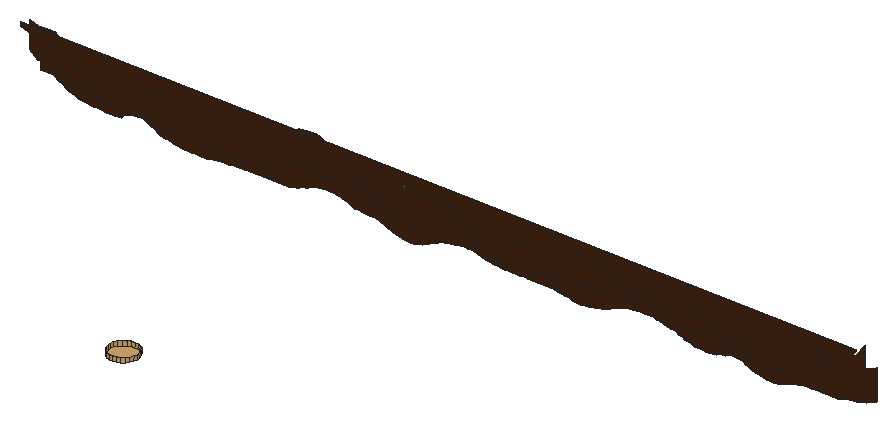
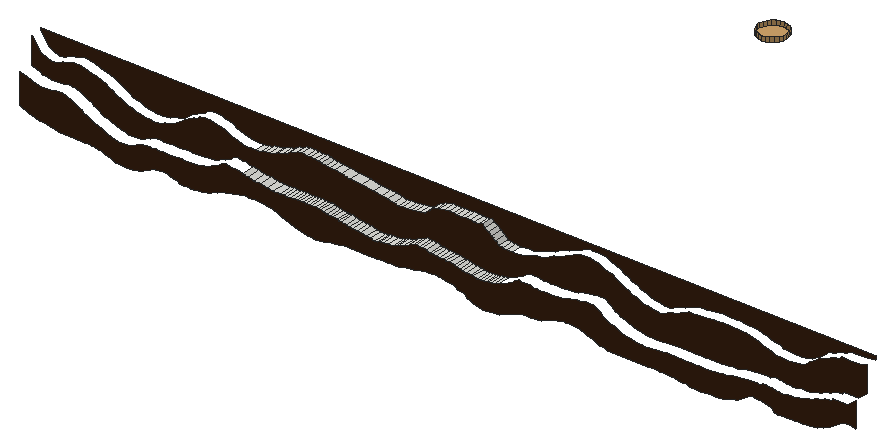
# SketchUp Ruby script. Lengths in inches.
U = 1.inch
M = Sketchup.active_model
def pt(a) = Geom::Point3d.new(a.map { |v| v * U })
def face(e, loops, mat)
  f = e.add_face(loops[0].map { |a| pt(a) })
  loops[1..].each { |l| e.add_face(l.map { |a| pt(a) }).erase! }
  f.material = f.back_material = mat if mat
  f
end
# faces: each face lists its corners as indices into pts; further lists are holes
def faces(e, pts, list, mat = nil) = list.each { |f| face(e, (f[0].is_a?(Array) ? f : [f]).map { |l| l.map { |i| pts[i] } }, mat) }
# xy, xz, yz: faces in a plane at the given z, y or x. An outline is a flat list of corners, or four numbers for a rectangle; further outlines are holes
def ring(l) = l.size == 4 ? [[l[0], l[1]], [l[2], l[1]], [l[2], l[3]], [l[0], l[3]]] : l.each_slice(2).to_a
def flat(e, list, mat, &to3) = list.each { |f| face(e, (f[0].is_a?(Array) ? f : [f]).map { |l| ring(l).map { |u, v| to3.(u, v) } }, mat) }
def xy(e, z, list, mat = nil) = flat(e, list, mat) { |x, y| [x, y, z] }
def xz(e, y, list, mat = nil) = flat(e, list, mat) { |x, z| [x, y, z] }
def yz(e, x, list, mat = nil) = flat(e, list, mat) { |y, z| [x, y, z] }
def lines(e, pts, list) = list.each { |a, b| e.add_line(pt(pts[a]), pt(pts[b])) }
# prism: a flat outline (further loops are holes) pulled along v
def prism(e, loops, v, mat = nil)
  f = face(e, loops, mat); d = Geom::Vector3d.new(v.map { |x| x * U })
  f.pushpull(f.normal.samedirection?(d) ? d.length : -d.length)
end
def box(e, o, s, mat = nil) = prism(e, [[o, [o[0] + s[0], o[1], o[2]], [o[0] + s[0], o[1] + s[1], o[2]], [o[0], o[1] + s[1], o[2]]]], [0, 0, s[2]], mat)
def at(x, y, z, deg = 0) = Geom::Transformation.translation(pt([x, y, z])) * Geom::Transformation.rotation(ORIGIN, Z_AXIS, deg.degrees)
def axes(o, x, y, z) = Geom::Transformation.new([*x, 0, *y, 0, *z, 0, *pt(o).to_a, 1])
def part(name) = M.definitions.add(name)
# library, detail: a bought-in or finely detailed component or shape, given as its bounding box
def library(name, o, s) = part(name).tap { |d| box(d.entities, o, s) }
def detail(e, o, s) = box(e.add_group.entities, o, s)
def put(e, d, t, mat = nil) = e.add_instance(d, t).tap { |i| i.material = mat if mat }
def group(e, t, mat = nil) = e.add_group.tap { |g| g.transformation = t; g.material = mat if mat }.entities
root = M.entities
M.materials.add("[Field Square Tile]").color = [211, 167, 108]
M.materials.add("[Wood Veneer 01]").color = [66, 38, 20]
xy(root,243.05,[[2115.79,2398.8,2116.47,2401.37]])
xy(root,243.07,[[2113.9375,2398.8,2114.52,2401.37]])
xy(root,243.09,[[2110.625,2398.8,2111.15,2401.37],[2111.15,2398.8,2111.67,2401.37],[2111.67,2398.8,2112.33,2401.37],[2112.33,2398.8,2112.78,2401.37]])
xy(root,249.21,[[2083.42,2396.68,2084.31,2398.8]])
xy(root,249.22,[[2085.03,2396.68,2085.9375,2398.8]])
xy(root,249.23,[[2086.58,2396.68,2087.48,2398.8]])
xy(root,250.6875,[[2081.97,2328.39,2081.31,2328.48,2080.69,2328.74,2080.16,2329.14,2079.75,2329.68,2079.5,2330.29,2079.41,2330.96,2079.5,2331.62,2079.75,2332.24,2080.16,2332.77,2080.69,2333.18,2081.31,2333.43,2081.97,2333.52,2082.63,2333.43,2083.25,2333.18,2083.78,2332.77,2084.19,2332.24,2084.45,2331.62,2084.53,2330.96,2084.45,2330.29,2084.19,2329.68,2083.78,2329.14,2083.25,2328.74,2082.63,2328.48]],"[Field Square Tile]")
xz(root,2396.68,[[2141.84,244.87,2142.75,245.01,2143.6875,245.12,2144.45,245.25,2145.21,245.41,2145.84,245.78,2146.64,245.88,2147.35,246.16,2147.95,246.57,2148.74,246.9,2149.34,247.35,2150.01,247.62,2150.6,248.06,2151.36,248.32,2152.47,248.66,2153.25,248.79,2154.11,249.19,2154.78,249.32,2155.71,249.41,2156.56,249.48,2157.31,249.21,2157.95,248.96,2158.65,248.9,2159.45,248.42,2160.16,248.3,2160.87,248.22,2161.6875,248.56,2162.62,249.02,2164.35,251.16,2164.35,251.5,2010.34,251.5,2010.34,250.88,2011.93,250.53,2013.55,250.54,2015.01,250.55,2015.54,250.15,2016.15,249.97,2016.95,249.8,2017.62,249.41,2018.29,249.2,2019.06,249.01,2019.55,248.51,2020.18,248.07,2020.83,247.72,2021.47,247.25,2022.02,246.88,2022.74,246.73,2023.4,246.62,2024.14,246.54,2024.92,246.51,2025.7,246.58,2026.5,246.59,2027.3,246.69,2028.01,247.03,2028.7,247.2,2029.67,247.39,2030.3,247.78,2031.08,247.89,2032.08,248.18,2032.72,248.29,2033.61,248.35,2034.34,248.4,2035.33,248.4375,2035.99,248.46,2036.88,248.47,2037.62,248.48,2038.51,248.49,2039.24,248.39,2040.64,248.28,2041.67,248.15,2042.49,248.11,2043.29,248.08,2044.13,247.66,2044.76,247.46,2045.44,247.08,2046.125,246.94,2046.98,246.66,2047.59,246.35,2048.36,246.05,2049.26,246.13,2049.97,246.29,2050.77,246.41,2051.68,246.55,2052.41,246.92,2053.02,247.12,2053.7,247.31,2054.27,247.71,2055.2,248.03,2055.91,248.46,2056.69,248.82,2057.41,249.37,2058.2,249.5625,2059.1,249.9,2060.02,250.35,2060.68,250.49,2061.49,250.6,2062.51,250.58,2063.15,250.61,2063.77,250.32,2064.46,250.0625,2065.12,249.68,2065.88,249.46,2066.77,248.95,2067.99,248.69,2068.9,248.26,2069.5,247.9,2070.63,247.66,2071.21,247.53,2071.89,247.25,2072.7,246.95,2073.39,246.75,2074.18,246.66,2074.89,246.59,2075.78,246.55,2076.71,246.63,2077.45,246.74,2078.18,246.87,2078.79,247.42,2079.46,247.96,2080.03,248.44,2080.77,248.85,2081.24,249.34,2081.97,249.125,2082.74,249.17,2083.42,249.21,2084.31,249.21,2085.03,249.22,2085.9375,249.22,2086.58,249.23,2087.48,249.23,2088.22,249.24,2089.02,249.14,2089.65,248.82,2090.44,248.54,2091.14,248.04,2091.83,247.48,2092.72,247.29,2093.54,247.15,2094.27,247.05,2094.99,247,2095.9,246.96,2096.625,246.94,2097.54,247.04,2098.6,247.36,2099.78,247.43,2101.43,247.6,2103.41,247.98,2105.61,248.1875,2107.22,248.49,2108.47,248.62,2109.41,248.69,2110.09,248.75,2110.75,249.09,2111.45,249.18,2112.23,249.13,2112.93,249.17,2113.63,249.18,2114.53,249.29,2115.26,249.21,2115.87,248.8,2116.5625,248.73,2117.34,248.26,2118.04,248.02,2118.84,247.8125,2119.55,247.4,2120.46,247.27,2121.2,247.18,2122.125,246.91,2122.99,246.84,2123.94,246.79,2124.72,246.75,2125.47,246.83,2126.51,247.25,2127.38,247.55,2128.05,247.66,2128.68,248.16,2129.47,248.41,2130.17,248.52,2130.87,248.72,2131.57,248.8,2132.46,248.85,2133.29,248.6875,2133.83,248.26,2134.52,248.06,2135.41,247.55,2136.12,247.19,2136.93,246.63,2137.5625,246.13,2138.15,245.83,2138.83,245.67,2139.7,245.46,2140.41,245.0625,2141.125,244.95]],"[Wood Veneer 01]")
xz(root,2398.8,[[2145.84,241.09,2146.41,241.14,2147.05,241.35,2147.64,241.46,2148.58,241.85,2149.58,242.23,2150.14,242.42,2150.86,242.61,2151.375,242.91,2151.75,243.14,2152.29,243.52,2152.77,243.71,2153.1,244.02,2153.54,244.21,2154.13,244.57,2154.6,244.76,2155.22,245.125,2155.72,245.32,2156.2,245.41,2156.75,245.48,2157.24,245.59,2157.77,245.55,2158.38,245.35,2158.87,245.31,2159.42,245.27,2159.98,245.24,2160.54,245.22,2161.1,245.34,2161.73,245.42,2162.3125,245.52,2162.69,245.76,2163.16,245.9,2164.35,246.43,2164.35,251.16,2162.62,249.02,2161.6875,248.56,2160.87,248.22,2160.16,248.3,2159.45,248.42,2158.65,248.9,2157.95,248.96,2157.31,249.21,2156.56,249.48,2155.71,249.41,2154.78,249.32,2154.11,249.19,2153.25,248.79,2152.47,248.66,2151.36,248.32,2150.6,248.06,2150.01,247.62,2149.34,247.35,2148.74,246.9,2147.95,246.57,2147.35,246.16,2146.64,245.88,2145.84,245.78,2145.21,245.41,2144.45,245.25,2143.6875,245.12,2142.75,245.01,2141.84,244.87,2141.125,244.95,2140.41,245.0625,2139.7,245.46,2138.83,245.67,2138.15,245.83,2137.5625,246.13,2136.93,246.63,2136.12,247.19,2135.41,247.55,2134.52,248.06,2133.83,248.26,2133.29,248.6875,2132.46,248.85,2131.57,248.8,2130.87,248.72,2130.17,248.52,2129.47,248.41,2128.68,248.16,2128.05,247.66,2127.38,247.55,2126.51,247.25,2125.47,246.83,2124.72,246.75,2123.94,246.79,2122.99,246.84,2122.125,246.91,2121.2,247.18,2120.46,247.27,2119.55,247.4,2118.84,247.8125,2118.04,248.02,2117.34,248.26,2116.5625,248.73,2115.87,248.8,2115.26,249.21,2114.53,249.29,2113.63,249.18,2112.93,249.17,2112.23,249.13,2111.45,249.18,2110.75,249.09,2110.09,248.75,2109.41,248.69,2108.47,248.62,2107.22,248.49,2105.61,248.1875,2103.41,247.98,2101.43,247.6,2099.78,247.43,2098.6,247.36,2097.54,247.04,2096.625,246.94,2095.9,246.96,2094.99,247,2094.27,247.05,2093.54,247.15,2092.72,247.29,2091.83,247.48,2091.14,248.04,2090.44,248.54,2089.65,248.82,2089.02,249.14,2088.22,249.24,2087.48,249.23,2086.58,249.23,2085.9375,249.22,2085.03,249.22,2084.31,249.21,2083.42,249.21,2082.74,249.17,2081.97,249.125,2081.24,249.34,2080.77,248.85,2080.03,248.44,2079.46,247.96,2078.79,247.42,2078.18,246.87,2077.45,246.74,2076.71,246.63,2075.78,246.55,2074.89,246.59,2074.18,246.66,2073.39,246.75,2072.7,246.95,2071.89,247.25,2071.21,247.53,2070.63,247.66,2069.5,247.9,2068.9,248.26,2067.99,248.69,2066.77,248.95,2065.88,249.46,2065.12,249.68,2064.46,250.0625,2063.77,250.32,2063.15,250.61,2062.51,250.58,2061.49,250.6,2060.68,250.49,2060.02,250.35,2059.1,249.9,2058.2,249.5625,2057.41,249.37,2056.69,248.82,2055.91,248.46,2055.2,248.03,2054.27,247.71,2053.7,247.31,2053.02,247.12,2052.41,246.92,2051.68,246.55,2050.77,246.41,2049.97,246.29,2049.26,246.13,2048.36,246.05,2047.59,246.35,2046.98,246.66,2046.125,246.94,2045.44,247.08,2044.76,247.46,2044.13,247.66,2043.29,248.08,2042.49,248.11,2041.67,248.15,2040.64,248.28,2039.24,248.39,2038.51,248.49,2037.62,248.48,2036.88,248.47,2035.99,248.46,2035.33,248.4375,2034.34,248.4,2033.61,248.35,2032.72,248.29,2032.08,248.18,2031.08,247.89,2030.3,247.78,2029.67,247.39,2028.7,247.2,2028.01,247.03,2027.3,246.69,2026.5,246.59,2025.7,246.58,2024.92,246.51,2024.14,246.54,2023.4,246.62,2022.74,246.73,2022.02,246.88,2021.47,247.25,2020.83,247.72,2020.18,248.07,2019.55,248.51,2019.06,249.01,2018.29,249.2,2017.62,249.41,2016.95,249.8,2016.15,249.97,2015.54,250.15,2015.01,250.55,2013.55,250.54,2011.93,250.53,2010.34,250.88,2010.34,246.2,2011.91,244.96,2013.3,244.9375,2014.55,244.92,2014.77,244.61,2015.33,244.54,2016.09,244.41,2016.76,244.11,2017.28,243.95,2017.94,243.79,2018.46,243.48,2019.1,243.3,2019.6875,243.14,2020.17,243.06,2020.89,242.85,2021.47,242.78,2022.28,242.73,2022.82,242.68,2023.49,242.51,2024.01,242.46,2024.55,242.58,2025.18,242.57,2025.81,242.81,2026.38,242.86,2026.94,242.89,2027.58,242.92,2028.01,242.625,2028.62,242.65,2029.17,242.62,2029.8,242.58,2030.36,242.57,2031,242.48,2031.66,242.38,2032.32,242.34,2032.99,242.24,2034.16,241.96,2034.93,241.89,2035.75,241.83,2036.35,241.78,2037.12,241.75,2037.57,241.74,2038.12,241.72,2039.38,241.7,2040.11,241.69,2040.78,241.68,2041.37,241.68,2041.86,241.67,2042.5625,241.74,2043.13,241.75,2045.13,241.75,2045.62,241.67,2046.15,241.66,2046.76,241.57,2047.3,241.53,2047.92,241.51,2048.47,241.49,2049.17,241.48,2049.83,241.47,2050.4,241.46,2051.11,241.6,2051.84,241.85,2052.51,241.91,2053.41,242.1,2054.18,242.46,2054.88,242.78,2055.65,242.97,2056.18,243.23,2056.58,243.48,2057.1,243.72,2057.4375,244.12,2057.91,244.39,2058.39,244.73,2058.875,244.87,2059.46,244.95,2060.14,245.01,2060.79,244.81,2061.36,244.7,2061.84,244.67,2062.45,244.55,2062.99,244.51,2063.45,244.25,2064.2,244.11,2064.76,244.04,2065.38,243.99,2066.1,243.95,2066.6,243.93,2067.29,243.91,2067.86,243.89,2068.56,243.88,2069.21,243.94,2069.85,243.95,2070.41,244.1,2071.04,244.13,2071.52,244.15,2072.04,244.17,2072.56,244.18,2073.16,243.8,2073.7,243.43,2074.31,243.09,2074.7,242.875,2075.2,242.68,2075.79,242.51,2076.3,242.21,2076.9,242.11,2077.58,241.96,2078.14,241.89,2078.6,241.85,2079.12,241.8125,2079.63,241.79,2080.21,241.78,2080.88,241.91,2081.35,241.93,2082.02,242.09,2082.79,242.2,2083.29,242.24,2083.9,242.42,2084.45,242.47,2085.2,242.71,2085.84,242.78,2086.32,242.82,2087.01,242.85,2087.71,242.87,2088.26,243.02,2088.88,243.05,2089.43,243.29,2090.11,243.35,2090.66,243.39,2091.26,243.42,2092.03,243.14,2092.6,242.9375,2093.15,242.65,2093.77,242.39,2094.53,242.14,2095.17,241.89,2095.66,241.78,2096.71,241.63,2097.48,241.56,2098.08,241.51,2098.53,241.48,2099.05,241.46,2099.92,241.51,2100.64,241.59,2101.58,241.82,2102.36,241.87,2103.125,241.98,2103.74,242.02,2104.39,242.19,2105.09,242.38,2105.58,242.4375,2106.1,242.48,2106.76,242.58,2107.29,242.61,2107.875,242.77,2108.33,242.95,2108.89,243.01,2109.4,243.05,2109.97,243.08,2110.625,243.09,2112.78,243.09,2113.35,243.08,2113.9375,243.07,2114.52,243.07,2115.18,243.0625,2115.79,243.05,2116.47,243.05,2117.74,243.1,2118.91,243.17,2120.05,243.4,2121.3125,243.52,2122.44,243.71,2123.34,243.99,2124.04,244.08,2124.74,244.21,2125.32,244.27,2125.86,244.3,2126.53,244.39,2127.125,244.19,2127.5,243.88,2127.98,243.59,2128.53,243.33,2129.08,243.22,2129.57,242.92,2130.05,242.75,2130.61,242.6,2131.17,242.52,2131.73,242.47,2132.3125,242.43,2132.89,242.4,2133.47,242.39,2134.05,242.37,2134.63,242.36,2135.22,242.35,2136.38,242.33,2136.96,242.33,2137.68,242.32,2138.15,242.3125,2138.79,242.3,2139.46,242.3,2139.91,242.29,2140.55,242.28,2141.0625,242.28,2141.69,242.2,2142.27,241.97,2142.84,241.84,2143.35,241.57,2143.77,241.33,2144.24,241.24,2144.77,241.17,2145.24,241.12]],"[Wood Veneer 01]")
xz(root,2401.37,[[2079.2,236.98,2079.88,237.22,2080.73,237.43,2081.35,237.74,2082.05,238.02,2082.49,238.375,2083.05,238.51,2083.6875,238.76,2084.33,239.12,2084.91,239.22,2085.91,239.31,2086.72,239.54,2087.21,239.6,2087.83,239.65,2088.42,239.69,2088.98,239.7,2089.71,239.72,2090.32,239.56,2090.99,239.44,2091.84,239.16,2092.39,239.07,2093.16,238.93,2094.04,238.78,2094.52,238.73,2095.19,238.6875,2095.88,238.66,2096.55,238.65,2097.33,238.64,2097.95,238.63,2098.64,238.625,2099.5,238.625,2100.06,238.62,2104.95,238.62,2105.64,238.45,2106.4,238.25,2107.02,238.19,2107.79,238.15,2108.42,237.86,2109.19,237.79,2109.9,237.74,2110.77,237.87,2111.42,237.88,2112.54,238.14,2113.76,238.46,2114.51,238.72,2115.39,239.08,2116.18,239.375,2116.92,239.75,2117.57,239.97,2118.19,240.17,2118.87,240.27,2119.55,240.33,2120.24,240.37,2120.93,240.4,2121.625,240.41,2122.15,240.42,2122.73,240.43,2123.3,240.43,2123.95,240.27,2124.53,240.23,2125.18,239.96,2125.9375,239.8,2126.55,239.65,2127.3125,239.5,2127.9375,239.18,2128.62,239.01,2129.14,238.67,2129.71,238.56,2130.37,238.48,2130.9375,238.26,2131.51,238.19,2132.33,238.15,2132.86,238.11,2133.53,238.18,2134.21,238.18,2134.89,238.27,2135.41,238.55,2136.07,238.61,2136.66,238.66,2137.23,239.04,2137.97,239.125,2138.65,239.02,2139.34,238.96,2139.86,238.86,2140.36,238.57,2140.91,238.33,2141.62,238,2142.45,237.71,2142.99,237.59,2143.59,237.51,2144.18,237.45,2144.75,237.42,2145.48,237.4,2146.16,237.47,2146.76,237.5625,2147.45,237.84,2148.13,238.08,2148.82,238.33,2149.35,238.51,2149.92,238.6,2150.58,238.74,2151.16,238.8,2151.73,238.83,2152.47,238.86,2153.23,238.875,2153.77,238.88,2154.45,238.89,2155.13,238.89,2155.89,238.9,2157.28,238.9,2157.91,239.15,2158.68,239.28,2159.48,239.42,2160.2,239.49,2160.75,239.53,2161.4375,239.81,2161.96,239.96,2162.52,240.1,2164.35,240.89,2164.35,246.43,2163.16,245.9,2162.69,245.76,2162.3125,245.52,2161.73,245.42,2161.1,245.34,2160.54,245.22,2159.98,245.24,2159.42,245.27,2158.87,245.31,2158.38,245.35,2157.77,245.55,2157.24,245.59,2156.75,245.48,2156.2,245.41,2155.72,245.32,2155.22,245.125,2154.6,244.76,2154.13,244.57,2153.54,244.21,2153.1,244.02,2152.77,243.71,2152.29,243.52,2151.75,243.14,2151.375,242.91,2150.86,242.61,2150.14,242.42,2149.58,242.23,2148.58,241.85,2147.64,241.46,2147.05,241.35,2146.41,241.14,2145.84,241.09,2145.24,241.12,2144.77,241.17,2144.24,241.24,2143.77,241.33,2143.35,241.57,2142.84,241.84,2142.27,241.97,2141.69,242.2,2141.0625,242.28,2140.55,242.28,2139.91,242.29,2139.46,242.3,2138.79,242.3,2138.15,242.3125,2137.68,242.32,2136.96,242.33,2136.38,242.33,2135.22,242.35,2134.63,242.36,2134.05,242.37,2133.47,242.39,2132.89,242.4,2132.3125,242.43,2131.73,242.47,2131.17,242.52,2130.61,242.6,2130.05,242.75,2129.57,242.92,2129.08,243.22,2128.53,243.33,2127.98,243.59,2127.5,243.88,2127.125,244.19,2126.53,244.39,2125.86,244.3,2125.32,244.27,2124.74,244.21,2124.04,244.08,2123.34,243.99,2122.44,243.71,2121.3125,243.52,2120.05,243.4,2118.91,243.17,2117.74,243.1,2116.47,243.05,2115.79,243.05,2115.18,243.0625,2114.52,243.07,2113.9375,243.07,2113.35,243.08,2112.78,243.09,2110.625,243.09,2109.97,243.08,2109.4,243.05,2108.89,243.01,2108.33,242.95,2107.875,242.77,2107.29,242.61,2106.76,242.58,2106.1,242.48,2105.58,242.4375,2105.09,242.38,2104.39,242.19,2103.74,242.02,2103.125,241.98,2102.36,241.87,2101.58,241.82,2100.64,241.59,2099.92,241.51,2099.05,241.46,2098.53,241.48,2098.08,241.51,2097.48,241.56,2096.71,241.63,2095.66,241.78,2095.17,241.89,2094.53,242.14,2093.77,242.39,2093.15,242.65,2092.6,242.9375,2092.03,243.14,2091.26,243.42,2090.66,243.39,2090.11,243.35,2089.43,243.29,2088.88,243.05,2088.26,243.02,2087.71,242.87,2087.01,242.85,2086.32,242.82,2085.84,242.78,2085.2,242.71,2084.45,242.47,2083.9,242.42,2083.29,242.24,2082.79,242.2,2082.02,242.09,2081.35,241.93,2080.88,241.91,2080.21,241.78,2079.63,241.79,2079.12,241.8125,2078.6,241.85,2078.14,241.89,2077.58,241.96,2076.9,242.11,2076.3,242.21,2075.79,242.51,2075.2,242.68,2074.7,242.875,2074.31,243.09,2073.7,243.43,2073.16,243.8,2072.56,244.18,2072.04,244.17,2071.52,244.15,2071.04,244.13,2070.41,244.1,2069.85,243.95,2069.21,243.94,2068.56,243.88,2067.86,243.89,2067.29,243.91,2066.6,243.93,2066.1,243.95,2065.38,243.99,2064.76,244.04,2064.2,244.11,2063.45,244.25,2062.99,244.51,2062.45,244.55,2061.84,244.67,2061.36,244.7,2060.79,244.81,2060.14,245.01,2059.46,244.95,2058.875,244.87,2058.39,244.73,2057.91,244.39,2057.4375,244.12,2057.1,243.72,2056.58,243.48,2056.18,243.23,2055.65,242.97,2054.88,242.78,2054.18,242.46,2053.41,242.1,2052.51,241.91,2051.84,241.85,2051.11,241.6,2050.4,241.46,2049.83,241.47,2049.17,241.48,2048.47,241.49,2047.92,241.51,2047.3,241.53,2046.76,241.57,2046.15,241.66,2045.62,241.67,2045.13,241.75,2043.13,241.75,2042.5625,241.74,2041.86,241.67,2041.37,241.68,2040.78,241.68,2040.11,241.69,2039.38,241.7,2038.12,241.72,2037.57,241.74,2037.12,241.75,2036.35,241.78,2035.75,241.83,2034.93,241.89,2034.16,241.96,2032.99,242.24,2032.32,242.34,2031.66,242.38,2031,242.48,2030.36,242.57,2029.8,242.58,2029.17,242.62,2028.62,242.65,2028.01,242.625,2027.58,242.92,2026.94,242.89,2026.38,242.86,2025.81,242.81,2025.18,242.57,2024.55,242.58,2024.01,242.46,2023.49,242.51,2022.82,242.68,2022.28,242.73,2021.47,242.78,2020.89,242.85,2020.17,243.06,2019.6875,243.14,2019.1,243.3,2018.46,243.48,2017.94,243.79,2017.28,243.95,2016.76,244.11,2016.09,244.41,2015.33,244.54,2014.77,244.61,2014.55,244.92,2013.3,244.9375,2011.91,244.96,2010.34,246.2,2010.34,241.52,2011.55,241.69,2012.82,241.55,2013.84,240.85,2014.38,240.59,2014.98,240.2,2015.77,239.86,2016.22,239.64,2016.78,239.52,2017.29,239.19,2018.07,239.09,2018.76,239.03,2019.44,238.97,2020.14,238.94,2020.84,238.93,2021.53,238.92,2022.57,238.82,2023.08,238.8,2023.95,238.79,2024.69,238.77,2025.22,238.9375,2025.78,239.55,2026.36,239.69,2026.91,239.88,2027.64,239.99,2028.23,240.05,2028.89,240.09,2029.58,240.11,2030.28,239.71,2030.74,239.38,2031.32,239.11,2031.9,238.74,2032.55,238.43,2033.46,238.31,2033.93,238.21,2034.87,237.9,2035.53,237.82,2036.22,237.76,2036.93,237.71,2037.54,237.68,2038.14,237.67,2038.89,237.66,2039.58,237.65,2040.89,237.65,2041.56,237.89,2042.32,237.94,2042.9375,237.98,2043.79,238.1,2044.34,238.13,2045.1,238.15,2045.73,238.26,2046.48,238.28,2047.11,238.3,2047.96,238.32,2048.68,238.33,2049.91,238.33,2050.59,238.34,2056.16,238.34,2056.67,238.59,2057.49,238.72,2058.18,238.86,2058.69,239.18,2059.28,239.35,2059.84,239.52,2060.39,239.85,2061.03,240.03,2061.6875,240.12,2062.36,240.19,2063.125,240.23,2063.83,240.25,2064.45,240.27,2065.23,240.11,2065.86,239.92,2066.55,239.7,2067.08,239.53,2067.66,239.29,2068.32,239.04,2068.9,238.94,2069.47,238.875,2070.22,238.83,2070.98,238.8,2071.52,238.79,2072.19,238.78,2072.97,238.43,2073.75,238.28,2074.3125,237.96,2075.25,237.68,2075.92,237.33,2076.45,237.2,2077.14,237.11,2077.9,237.04,2078.59,237.01]],"[Wood Veneer 01]")
p = [[2097.48,2398.8,241.56],[2097.48,2401.37,241.56],[2098.08,2401.37,241.51],[2098.08,2398.8,241.51],[2098.53,2401.37,241.48],[2098.53,2398.8,241.48],
  [2099.05,2401.37,241.46],[2099.05,2398.8,241.46],[2099.92,2401.37,241.51],[2099.92,2398.8,241.51],[2100.64,2401.37,241.59],[2100.64,2398.8,241.59],
  [2095.66,2398.8,241.78],[2095.66,2401.37,241.78],[2096.71,2401.37,241.63],[2096.71,2398.8,241.63],[2101.58,2401.37,241.82],[2101.58,2398.8,241.82],
  [2078.14,2398.8,241.89],[2078.14,2401.37,241.89],[2078.6,2401.37,241.85],[2078.6,2398.8,241.85],[2079.12,2401.37,241.8125],[2079.12,2398.8,241.8125],
  [2079.63,2401.37,241.79],[2079.63,2398.8,241.79],[2080.21,2401.37,241.78],[2080.21,2398.8,241.78],[2080.88,2401.37,241.91],[2080.88,2398.8,241.91],
  [2095.17,2398.8,241.89],[2095.17,2401.37,241.89],[2102.36,2401.37,241.87],[2102.36,2398.8,241.87],[2077.58,2398.8,241.96],[2077.58,2401.37,241.96],
  [2081.35,2401.37,241.93],[2081.35,2398.8,241.93],[2082.02,2401.37,242.09],[2082.02,2398.8,242.09],[2094.53,2398.8,242.14],[2094.53,2401.37,242.14],
  [2103.125,2401.37,241.98],[2103.125,2398.8,241.98],[2076.9,2398.8,242.11],[2076.9,2401.37,242.11],[2103.74,2401.37,242.02],[2103.74,2398.8,242.02],
  [2104.39,2401.37,242.19],[2104.39,2398.8,242.19],[2076.3,2398.8,242.21],[2076.3,2401.37,242.21],[2082.79,2401.37,242.2],[2082.79,2398.8,242.2],
  [2093.77,2398.8,242.39],[2093.77,2401.37,242.39],[2083.29,2401.37,242.24],[2083.29,2398.8,242.24],[2083.9,2401.37,242.42],[2083.9,2398.8,242.42],
  [2105.09,2401.37,242.38],[2105.09,2398.8,242.38],[2084.45,2401.37,242.47],[2084.45,2398.8,242.47],[2093.15,2398.8,242.65],[2093.15,2401.37,242.65],
  [2105.58,2401.37,242.4375],[2105.58,2398.8,242.4375],[2106.1,2401.37,242.48],[2106.1,2398.8,242.48],[2085.2,2401.37,242.71],[2085.2,2398.8,242.71],
  [2106.76,2401.37,242.58],[2106.76,2398.8,242.58],[2092.6,2398.8,242.9375],[2092.6,2401.37,242.9375],[2107.29,2401.37,242.61],[2107.29,2398.8,242.61],
  [2107.875,2401.37,242.77],[2107.875,2398.8,242.77],[2085.84,2401.37,242.78],[2085.84,2398.8,242.78],[2086.32,2401.37,242.82],[2086.32,2398.8,242.82],
  [2087.01,2401.37,242.85],[2087.01,2398.8,242.85],[2108.33,2401.37,242.95],[2108.33,2398.8,242.95],[2087.71,2401.37,242.87],[2087.71,2398.8,242.87],
  [2088.26,2401.37,243.02],[2088.26,2398.8,243.02],[2092.03,2398.8,243.14],[2092.03,2401.37,243.14],[2088.88,2401.37,243.05],[2088.88,2398.8,243.05],
  [2108.89,2401.37,243.01],[2108.89,2398.8,243.01],[2109.4,2401.37,243.05],[2109.4,2398.8,243.05],[2109.97,2401.37,243.08],[2109.97,2398.8,243.08],
  [2116.47,2398.8,243.05],[2116.47,2401.37,243.05],[2117.74,2401.37,243.1],[2117.74,2398.8,243.1],[2089.43,2401.37,243.29],[2089.43,2398.8,243.29],
  [2091.26,2398.8,243.42],[2091.26,2401.37,243.42],[2110.625,2401.37,243.09],[2110.625,2398.8,243.09],[2112.78,2398.8,243.09],[2112.78,2401.37,243.09],
  [2113.35,2401.37,243.08],[2113.35,2398.8,243.08],[2113.9375,2401.37,243.07],[2113.9375,2398.8,243.07],[2114.52,2398.8,243.07],[2114.52,2401.37,243.07],
  [2115.18,2401.37,243.0625],[2115.18,2398.8,243.0625],[2115.79,2401.37,243.05],[2115.79,2398.8,243.05],[2118.91,2401.37,243.17],[2118.91,2398.8,243.17],
  [2120.05,2401.37,243.4],[2120.05,2398.8,243.4],[2090.11,2401.37,243.35],[2090.11,2398.8,243.35],[2090.66,2401.37,243.39],[2090.66,2398.8,243.39],
  [2121.3125,2401.37,243.52],[2121.3125,2398.8,243.52],[2122.44,2401.37,243.71],[2122.44,2398.8,243.71],[2123.34,2401.37,243.99],[2123.34,2398.8,243.99],
  [2075.78,2396.68,246.55],[2075.78,2398.8,246.55],[2076.71,2398.8,246.63],[2076.71,2396.68,246.63],[2077.45,2398.8,246.74],[2077.45,2396.68,246.74],
  [2078.18,2398.8,246.87],[2078.18,2396.68,246.87],[2122.125,2396.68,246.91],[2122.125,2398.8,246.91],[2122.99,2398.8,246.84],[2122.99,2396.68,246.84],
  [2078.79,2398.8,247.42],[2078.79,2396.68,247.42],[2095.9,2396.68,246.96],[2095.9,2398.8,246.96],[2096.625,2398.8,246.94],[2096.625,2396.68,246.94],
  [2097.54,2398.8,247.04],[2097.54,2396.68,247.04],[2121.2,2396.68,247.18],[2121.2,2398.8,247.18],[2093.54,2396.68,247.15],[2093.54,2398.8,247.15],
  [2094.27,2398.8,247.05],[2094.27,2396.68,247.05],[2094.99,2398.8,247],[2094.99,2396.68,247],[2098.6,2398.8,247.36],[2098.6,2396.68,247.36],
  [2092.72,2396.68,247.29],[2092.72,2398.8,247.29],[2120.46,2396.68,247.27],[2120.46,2398.8,247.27],[2091.83,2396.68,247.48],[2091.83,2398.8,247.48],
  [2119.55,2396.68,247.4],[2119.55,2398.8,247.4],[2079.46,2398.8,247.96],[2079.46,2396.68,247.96],[2099.78,2398.8,247.43],[2099.78,2396.68,247.43],
  [2101.43,2398.8,247.6],[2101.43,2396.68,247.6],[2118.84,2396.68,247.8125],[2118.84,2398.8,247.8125],[2091.14,2396.68,248.04],[2091.14,2398.8,248.04],
  [2103.41,2398.8,247.98],[2103.41,2396.68,247.98],[2118.04,2396.68,248.02],[2118.04,2398.8,248.02],[2080.03,2398.8,248.44],[2080.03,2396.68,248.44],
  [2090.44,2396.68,248.54],[2090.44,2398.8,248.54],[2105.61,2398.8,248.1875],[2105.61,2396.68,248.1875],[2117.34,2396.68,248.26],[2117.34,2398.8,248.26],
  [2107.22,2398.8,248.49],[2107.22,2396.68,248.49],[2116.5625,2396.68,248.73],[2116.5625,2398.8,248.73],[2080.77,2398.8,248.85],[2080.77,2396.68,248.85],
  [2089.65,2396.68,248.82],[2089.65,2398.8,248.82],[2108.47,2398.8,248.62],[2108.47,2396.68,248.62],[2109.41,2398.8,248.69],[2109.41,2396.68,248.69],
  [2110.09,2398.8,248.75],[2110.09,2396.68,248.75],[2115.87,2396.68,248.8],[2115.87,2398.8,248.8],[2089.02,2396.68,249.14],[2089.02,2398.8,249.14],
  [2110.75,2398.8,249.09],[2110.75,2396.68,249.09],[2115.26,2396.68,249.21],[2115.26,2398.8,249.21],[2081.24,2398.8,249.34],[2081.24,2396.68,249.34],
  [2081.97,2398.8,249.125],[2081.97,2396.68,249.125],[2082.74,2398.8,249.17],[2082.74,2396.68,249.17],[2088.22,2396.68,249.24],[2088.22,2398.8,249.24],
  [2111.45,2398.8,249.18],[2111.45,2396.68,249.18],[2112.23,2398.8,249.13],[2112.23,2396.68,249.13],[2112.93,2398.8,249.17],[2112.93,2396.68,249.17],
  [2083.42,2398.8,249.21],[2083.42,2396.68,249.21],[2084.31,2396.68,249.21],[2084.31,2398.8,249.21],[2085.03,2398.8,249.22],[2085.03,2396.68,249.22],
  [2085.9375,2396.68,249.22],[2085.9375,2398.8,249.22],[2086.58,2398.8,249.23],[2086.58,2396.68,249.23],[2087.48,2396.68,249.23],[2087.48,2398.8,249.23],
  [2113.63,2398.8,249.18],[2113.63,2396.68,249.18],[2114.53,2398.8,249.29],[2114.53,2396.68,249.29],[2081.97,2328.39,251.5],[2081.31,2328.48,251.5],
  [2081.31,2328.48,250.6875],[2081.97,2328.39,250.6875],[2082.63,2328.48,251.5],[2082.63,2328.48,250.6875],[2080.69,2328.74,251.5],[2080.69,2328.74,250.6875],
  [2083.25,2328.74,251.5],[2083.25,2328.74,250.6875],[2080.16,2329.14,251.5],[2080.16,2329.14,250.6875],[2083.78,2329.14,251.5],[2083.78,2329.14,250.6875],
  [2079.75,2329.68,251.5],[2079.75,2329.68,250.6875],[2084.19,2329.68,251.5],[2084.19,2329.68,250.6875],[2079.5,2330.29,251.5],[2079.5,2330.29,250.6875],
  [2084.45,2330.29,251.5],[2084.45,2330.29,250.6875],[2079.41,2330.96,251.5],[2079.41,2330.96,250.6875],[2084.53,2330.96,251.5],[2084.53,2330.96,250.6875],
  [2079.5,2331.62,251.5],[2079.5,2331.62,250.6875],[2084.45,2331.62,251.5],[2084.45,2331.62,250.6875],[2079.75,2332.24,251.5],[2079.75,2332.24,250.6875],
  [2084.19,2332.24,251.5],[2084.19,2332.24,250.6875],[2080.16,2332.77,251.5],[2080.16,2332.77,250.6875],[2083.78,2332.77,251.5],[2083.78,2332.77,250.6875],
  [2080.69,2333.18,251.5],[2080.69,2333.18,250.6875],[2083.25,2333.18,251.5],[2083.25,2333.18,250.6875],[2081.31,2333.43,251.5],[2081.31,2333.43,250.6875],
  [2082.63,2333.43,251.5],[2082.63,2333.43,250.6875],[2081.97,2333.52,251.5],[2081.97,2333.52,250.6875]]
faces(root,p,[[0,1,2,3],[3,2,4,5],[5,4,6,7],[7,6,8,9],[9,8,10,11],[12,13,14,15],[15,14,1,0],[11,10,16,17],
  [18,19,20,21],[21,20,22,23],[23,22,24,25],[25,24,26,27],[27,26,28,29],[30,31,13,12],[17,16,32,33],[34,35,19,18],
  [29,28,36,37],[37,36,38,39],[40,41,31,30],[33,32,42,43],[44,45,35,34],[43,42,46,47],[47,46,48,49],[50,51,45,44],
  [39,38,52,53],[54,55,41,40],[53,52,56,57],[57,56,58,59],[49,48,60,61],[59,58,62,63],[64,65,55,54],[61,60,66,67],
  [67,66,68,69],[63,62,70,71],[69,68,72,73],[74,75,65,64],[73,72,76,77],[77,76,78,79],[71,70,80,81],[81,80,82,83],
  [83,82,84,85],[79,78,86,87],[85,84,88,89],[89,88,90,91],[92,93,75,74],[91,90,94,95],[87,86,96,97],[97,96,98,99],
  [99,98,100,101],[102,103,104,105],[95,94,106,107],[108,109,93,92],[101,100,110,111],[112,113,114,115],[115,114,116,117],[118,119,120,121],
  [121,120,122,123],[105,104,124,125],[125,124,126,127],[107,106,128,129],[129,128,130,131],[131,130,109,108],[127,126,132,133],[133,132,134,135],
  [135,134,136,137],[138,139,140,141],[141,140,142,143],[143,142,144,145],[146,147,148,149],[145,144,150,151],[152,153,154,155],[155,154,156,157],
  [158,159,147,146],[160,161,162,163],[163,162,164,165],[165,164,153,152],[157,156,166,167],[168,169,161,160],[170,171,159,158],[172,173,169,168],
  [174,175,171,170],[151,150,176,177],[167,166,178,179],[179,178,180,181],[182,183,175,174],[184,185,173,172],[181,180,186,187],[188,189,183,182],
  [177,176,190,191],[192,193,185,184],[187,186,194,195],[196,197,189,188],[195,194,198,199],[200,201,197,196],[191,190,202,203],[204,205,193,192],
  [199,198,206,207],[207,206,208,209],[209,208,210,211],[212,213,201,200],[214,215,205,204],[211,210,216,217],[218,219,213,212],[203,202,220,221],
  [221,220,222,223],[223,222,224,225],[226,227,215,214],[217,216,228,229],[229,228,230,231],[231,230,232,233],[225,224,234,235],[236,237,238,239],
  [240,241,242,243],[244,245,227,226],[233,232,246,247],[247,246,248,249],[249,248,219,218]])
faces(root,p,[[250,251,252,253],[254,250,253,255],[251,256,257,252],[258,254,255,259],[256,260,261,257],[262,258,259,263],[260,264,265,261],[266,262,263,267],
  [264,268,269,265],[270,266,267,271],[268,272,273,269],[274,270,271,275],[272,276,277,273],[278,274,275,279],[276,280,281,277],[282,278,279,283],
  [280,284,285,281],[286,282,283,287],[284,288,289,285],[290,286,287,291],[288,292,293,289],[294,290,291,295],[292,296,297,293],[296,294,295,297]],"[Field Square Tile]")
